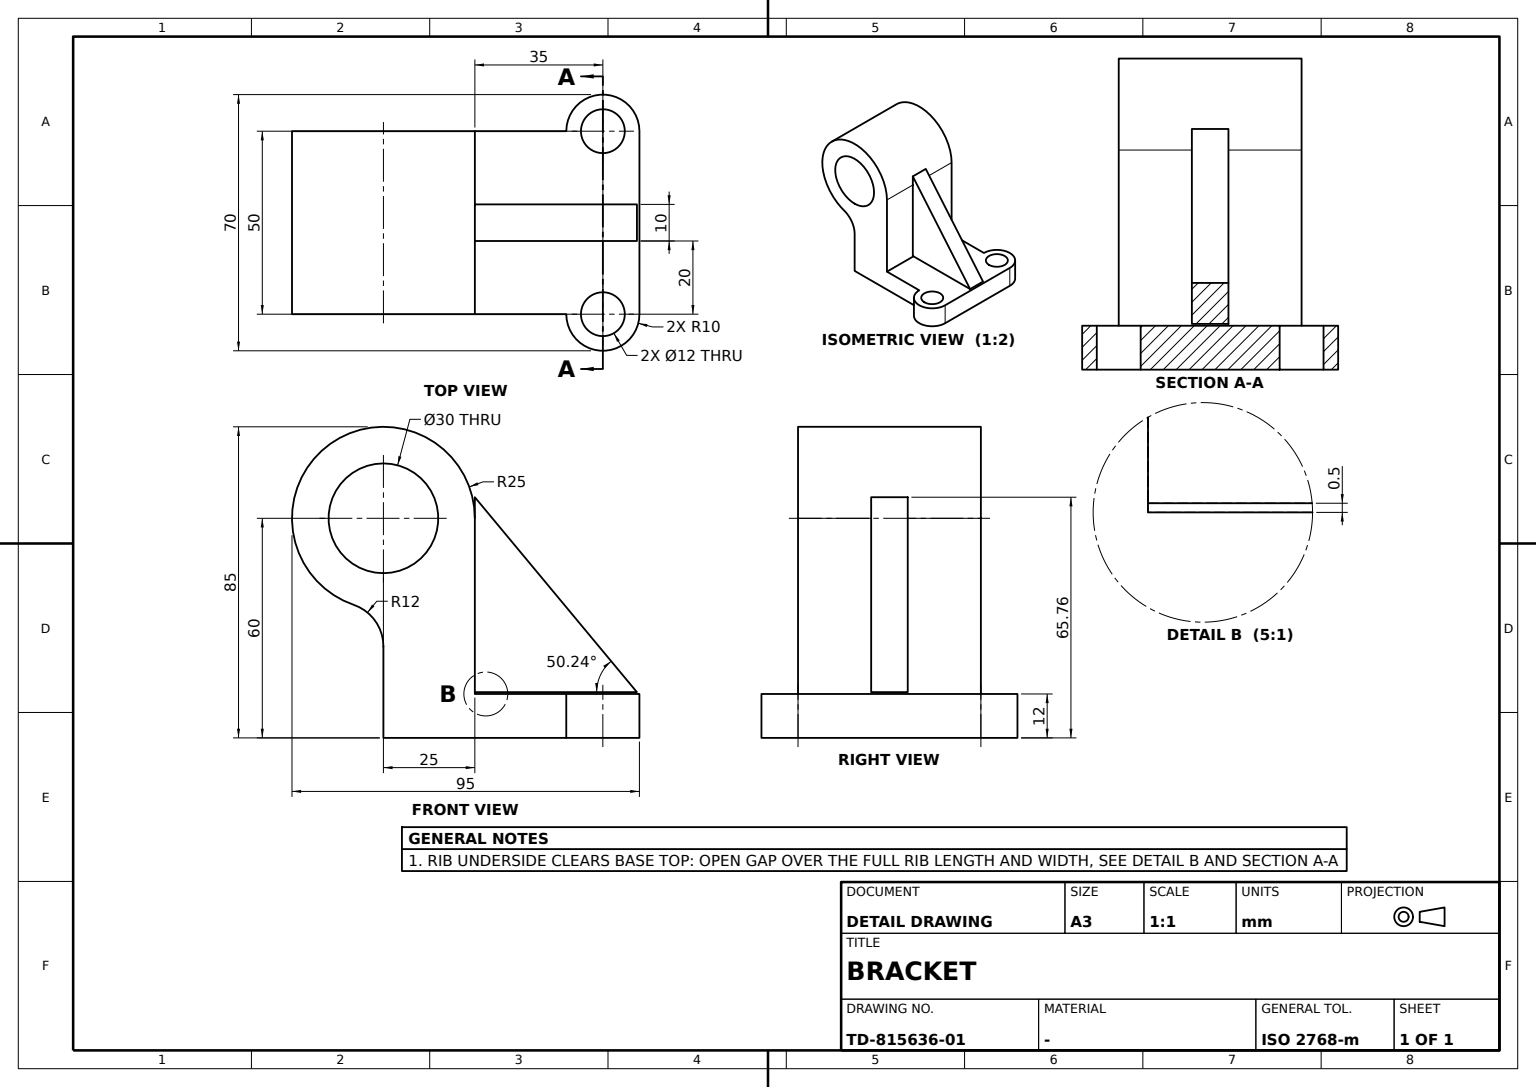
ISO-10303-21;
HEADER;
FILE_DESCRIPTION((''),'2;1');
FILE_NAME('','',(''),(''),'','','');
FILE_SCHEMA(('AUTOMOTIVE_DESIGN'));
ENDSEC;
DATA;
#1=APPLICATION_CONTEXT('');
#2=PRODUCT_CONTEXT('',#1,'mechanical');
#3=PRODUCT('','','',(#2));
#4=PRODUCT_DEFINITION_FORMATION('','',#3);
#5=PRODUCT_DEFINITION_CONTEXT('',#1,'design');
#6=PRODUCT_DEFINITION('','',#4,#5);
#7=PRODUCT_DEFINITION_SHAPE('','',#6);
#8=(LENGTH_UNIT()NAMED_UNIT(*)SI_UNIT(.MILLI.,.METRE.));
#9=(NAMED_UNIT(*)PLANE_ANGLE_UNIT()SI_UNIT($,.RADIAN.));
#10=(NAMED_UNIT(*)SI_UNIT($,.STERADIAN.)SOLID_ANGLE_UNIT());
#11=UNCERTAINTY_MEASURE_WITH_UNIT(LENGTH_MEASURE(0.005),#8,'distance_accuracy_value','');
#12=(GEOMETRIC_REPRESENTATION_CONTEXT(3)GLOBAL_UNCERTAINTY_ASSIGNED_CONTEXT((#11))GLOBAL_UNIT_ASSIGNED_CONTEXT((#8,#9,#10))REPRESENTATION_CONTEXT('',''));
#13=CARTESIAN_POINT('',(20.,0.,6.5));
#14=VERTEX_POINT('',#13);
#15=CARTESIAN_POINT('',(20.,44.314968,6.5));
#16=VERTEX_POINT('',#15);
#17=DIRECTION('',(0.,1.,0.));
#18=VECTOR('',#17,1000.);
#19=LINE('',#13,#18);
#20=EDGE_CURVE('',#14,#16,#19,.T.);
#21=ORIENTED_EDGE('',*,*,#20,.F.);
#22=CARTESIAN_POINT('',(20.,0.,54.));
#23=VERTEX_POINT('',#22);
#24=CARTESIAN_POINT('',(20.,0.,0.));
#25=DIRECTION('',(0.,0.,-1.));
#26=VECTOR('',#25,1000.);
#27=LINE('',#24,#26);
#28=EDGE_CURVE('',#23,#14,#27,.T.);
#29=ORIENTED_EDGE('',*,*,#28,.F.);
#30=CARTESIAN_POINT('',(20.,0.,59.759468));
#31=VERTEX_POINT('',#30);
#32=EDGE_CURVE('',#31,#23,#27,.T.);
#33=ORIENTED_EDGE('',*,*,#32,.F.);
#34=CARTESIAN_POINT('',(20.,29.381753,24.447324));
#35=DIRECTION('',(0.,-0.639605663,0.768703191));
#36=VECTOR('',#35,1000.);
#37=LINE('',#34,#36);
#38=EDGE_CURVE('',#16,#31,#37,.T.);
#39=ORIENTED_EDGE('',*,*,#38,.F.);
#40=EDGE_LOOP('',(#21,#29,#33,#39));
#41=FACE_BOUND('',#40,.T.);
#42=DIRECTION('',(1.,0.,0.));
#43=AXIS2_PLACEMENT_3D('',#24,#42,#17);
#44=PLANE('',#43);
#45=ADVANCED_FACE('',(#41),#44,.F.);
#46=CARTESIAN_POINT('',(0.,-25.,39.));
#47=VERTEX_POINT('',#46);
#48=CARTESIAN_POINT('',(0.,-25.,54.));
#49=AXIS2_PLACEMENT_3D('',#48,#42,#25);
#50=CIRCLE('',#49,15.);
#51=EDGE_CURVE('',#47,#47,#50,.T.);
#52=ORIENTED_EDGE('',*,*,#51,.T.);
#53=EDGE_LOOP('',(#52));
#54=FACE_BOUND('',#53,.T.);
#55=CARTESIAN_POINT('',(0.,-25.,19.));
#56=VERTEX_POINT('',#55);
#57=CARTESIAN_POINT('',(0.,-33.108108,30.351351));
#58=VERTEX_POINT('',#57);
#59=CARTESIAN_POINT('',(0.,-37.,19.));
#60=AXIS2_PLACEMENT_3D('',#59,#42,#25);
#61=CIRCLE('',#60,12.);
#62=EDGE_CURVE('',#56,#58,#61,.T.);
#63=ORIENTED_EDGE('',*,*,#62,.T.);
#64=CARTESIAN_POINT('',(0.,0.,54.));
#65=VERTEX_POINT('',#64);
#66=CIRCLE('',#49,25.);
#67=EDGE_CURVE('',#65,#58,#66,.T.);
#68=ORIENTED_EDGE('',*,*,#67,.F.);
#69=CARTESIAN_POINT('',(0.,0.,6.));
#70=VERTEX_POINT('',#69);
#71=CARTESIAN_POINT('',(0.,0.,0.));
#72=LINE('',#71,#26);
#73=EDGE_CURVE('',#65,#70,#72,.T.);
#74=ORIENTED_EDGE('',*,*,#73,.T.);
#75=CARTESIAN_POINT('',(0.,25.,6.));
#76=VERTEX_POINT('',#75);
#77=LINE('',#69,#18);
#78=EDGE_CURVE('',#70,#76,#77,.T.);
#79=ORIENTED_EDGE('',*,*,#78,.T.);
#80=CARTESIAN_POINT('',(0.,25.,-6.));
#81=VERTEX_POINT('',#80);
#82=DIRECTION('',(0.,0.,1.));
#83=VECTOR('',#82,1000.);
#84=LINE('',#80,#83);
#85=EDGE_CURVE('',#81,#76,#84,.T.);
#86=ORIENTED_EDGE('',*,*,#85,.F.);
#87=CARTESIAN_POINT('',(0.,-25.,-6.));
#88=VERTEX_POINT('',#87);
#89=CARTESIAN_POINT('',(0.,0.,-6.));
#90=DIRECTION('',(0.,-1.,0.));
#91=VECTOR('',#90,1000.);
#92=LINE('',#89,#91);
#93=EDGE_CURVE('',#81,#88,#92,.T.);
#94=ORIENTED_EDGE('',*,*,#93,.T.);
#95=CARTESIAN_POINT('',(0.,-25.,0.));
#96=LINE('',#95,#83);
#97=EDGE_CURVE('',#88,#56,#96,.T.);
#98=ORIENTED_EDGE('',*,*,#97,.T.);
#99=EDGE_LOOP('',(#63,#68,#74,#79,#86,#94,#98));
#100=FACE_BOUND('',#99,.T.);
#101=AXIS2_PLACEMENT_3D('',#71,#42,#17);
#102=PLANE('',#101);
#103=ADVANCED_FACE('',(#54,#100),#102,.F.);
#104=CARTESIAN_POINT('',(50.,-25.,39.));
#105=VERTEX_POINT('',#104);
#106=CARTESIAN_POINT('',(50.,-25.,54.));
#107=AXIS2_PLACEMENT_3D('',#106,#42,#25);
#108=CIRCLE('',#107,15.);
#109=EDGE_CURVE('',#105,#105,#108,.T.);
#110=ORIENTED_EDGE('',*,*,#109,.T.);
#111=EDGE_LOOP('',(#110));
#112=FACE_BOUND('',#111,.T.);
#113=ORIENTED_EDGE('',*,*,#51,.F.);
#114=EDGE_LOOP('',(#113));
#115=FACE_BOUND('',#114,.T.);
#116=CARTESIAN_POINT('',(25.,-25.,54.));
#117=AXIS2_PLACEMENT_3D('',#116,#42,#17);
#118=CYLINDRICAL_SURFACE('',#117,15.);
#119=ADVANCED_FACE('',(#112,#115),#118,.F.);
#120=CARTESIAN_POINT('',(6.,35.,-6.));
#121=VERTEX_POINT('',#120);
#122=CARTESIAN_POINT('',(0.,35.,-6.));
#123=AXIS2_PLACEMENT_3D('',#122,#82,#42);
#124=CIRCLE('',#123,6.);
#125=EDGE_CURVE('',#121,#121,#124,.T.);
#126=ORIENTED_EDGE('',*,*,#125,.F.);
#127=EDGE_LOOP('',(#126));
#128=FACE_BOUND('',#127,.T.);
#129=CARTESIAN_POINT('',(-6.,35.,6.));
#130=VERTEX_POINT('',#129);
#131=CARTESIAN_POINT('',(0.,35.,6.));
#132=DIRECTION('',(-1.,0.,0.));
#133=AXIS2_PLACEMENT_3D('',#131,#25,#132);
#134=CIRCLE('',#133,6.);
#135=EDGE_CURVE('',#130,#130,#134,.F.);
#136=ORIENTED_EDGE('',*,*,#135,.T.);
#137=EDGE_LOOP('',(#136));
#138=FACE_BOUND('',#137,.T.);
#139=CARTESIAN_POINT('',(0.,35.,0.));
#140=AXIS2_PLACEMENT_3D('',#139,#82,#42);
#141=CYLINDRICAL_SURFACE('',#140,6.);
#142=ADVANCED_FACE('',(#128,#138),#141,.F.);
#143=CARTESIAN_POINT('',(50.,-25.,19.));
#144=VERTEX_POINT('',#143);
#145=CARTESIAN_POINT('',(50.,-33.108108,30.351351));
#146=VERTEX_POINT('',#145);
#147=CARTESIAN_POINT('',(50.,-37.,19.));
#148=AXIS2_PLACEMENT_3D('',#147,#42,#25);
#149=CIRCLE('',#148,12.);
#150=EDGE_CURVE('',#144,#146,#149,.T.);
#151=ORIENTED_EDGE('',*,*,#150,.T.);
#152=CARTESIAN_POINT('',(25.,-33.108108,30.351351));
#153=VECTOR('',#42,1000.);
#154=LINE('',#152,#153);
#155=EDGE_CURVE('',#58,#146,#154,.T.);
#156=ORIENTED_EDGE('',*,*,#155,.F.);
#157=ORIENTED_EDGE('',*,*,#62,.F.);
#158=CARTESIAN_POINT('',(25.,-25.,19.));
#159=LINE('',#158,#153);
#160=EDGE_CURVE('',#56,#144,#159,.T.);
#161=ORIENTED_EDGE('',*,*,#160,.T.);
#162=EDGE_LOOP('',(#151,#156,#157,#161));
#163=FACE_BOUND('',#162,.T.);
#164=CARTESIAN_POINT('',(25.,-37.,19.));
#165=AXIS2_PLACEMENT_3D('',#164,#42,#17);
#166=CYLINDRICAL_SURFACE('',#165,12.);
#167=ADVANCED_FACE('',(#163),#166,.F.);
#168=CARTESIAN_POINT('',(30.,44.314968,6.5));
#169=VERTEX_POINT('',#168);
#170=CARTESIAN_POINT('',(30.,0.,59.759468));
#171=VERTEX_POINT('',#170);
#172=CARTESIAN_POINT('',(30.,29.381753,24.447324));
#173=LINE('',#172,#36);
#174=EDGE_CURVE('',#169,#171,#173,.T.);
#175=ORIENTED_EDGE('',*,*,#174,.T.);
#176=CARTESIAN_POINT('',(30.,0.,54.));
#177=VERTEX_POINT('',#176);
#178=CARTESIAN_POINT('',(30.,0.,0.));
#179=LINE('',#178,#26);
#180=EDGE_CURVE('',#171,#177,#179,.T.);
#181=ORIENTED_EDGE('',*,*,#180,.T.);
#182=CARTESIAN_POINT('',(30.,0.,6.5));
#183=VERTEX_POINT('',#182);
#184=EDGE_CURVE('',#177,#183,#179,.T.);
#185=ORIENTED_EDGE('',*,*,#184,.T.);
#186=LINE('',#182,#18);
#187=EDGE_CURVE('',#183,#169,#186,.T.);
#188=ORIENTED_EDGE('',*,*,#187,.T.);
#189=EDGE_LOOP('',(#175,#181,#185,#188));
#190=FACE_BOUND('',#189,.T.);
#191=AXIS2_PLACEMENT_3D('',#178,#42,#17);
#192=PLANE('',#191);
#193=ADVANCED_FACE('',(#190),#192,.T.);
#194=CARTESIAN_POINT('',(44.,35.,6.));
#195=VERTEX_POINT('',#194);
#196=CARTESIAN_POINT('',(50.,35.,6.));
#197=AXIS2_PLACEMENT_3D('',#196,#25,#132);
#198=CIRCLE('',#197,6.);
#199=EDGE_CURVE('',#195,#195,#198,.F.);
#200=ORIENTED_EDGE('',*,*,#199,.T.);
#201=EDGE_LOOP('',(#200));
#202=FACE_BOUND('',#201,.T.);
#203=CARTESIAN_POINT('',(56.,35.,-6.));
#204=VERTEX_POINT('',#203);
#205=CARTESIAN_POINT('',(50.,35.,-6.));
#206=AXIS2_PLACEMENT_3D('',#205,#82,#42);
#207=CIRCLE('',#206,6.);
#208=EDGE_CURVE('',#204,#204,#207,.T.);
#209=ORIENTED_EDGE('',*,*,#208,.F.);
#210=EDGE_LOOP('',(#209));
#211=FACE_BOUND('',#210,.T.);
#212=CARTESIAN_POINT('',(50.,35.,0.));
#213=AXIS2_PLACEMENT_3D('',#212,#82,#42);
#214=CYLINDRICAL_SURFACE('',#213,6.);
#215=ADVANCED_FACE('',(#202,#211),#214,.F.);
#216=CARTESIAN_POINT('',(25.,44.314968,6.5));
#217=LINE('',#216,#153);
#218=EDGE_CURVE('',#16,#169,#217,.T.);
#219=ORIENTED_EDGE('',*,*,#218,.F.);
#220=ORIENTED_EDGE('',*,*,#38,.T.);
#221=CARTESIAN_POINT('',(25.,0.,59.759468));
#222=LINE('',#221,#153);
#223=EDGE_CURVE('',#31,#171,#222,.T.);
#224=ORIENTED_EDGE('',*,*,#223,.T.);
#225=ORIENTED_EDGE('',*,*,#174,.F.);
#226=EDGE_LOOP('',(#219,#220,#224,#225));
#227=FACE_BOUND('',#226,.T.);
#228=DIRECTION('',(0.,0.768703191,0.639605663));
#229=AXIS2_PLACEMENT_3D('',#216,#228,#35);
#230=PLANE('',#229);
#231=ADVANCED_FACE('',(#227),#230,.T.);
#232=CARTESIAN_POINT('',(50.,25.,-6.));
#233=VERTEX_POINT('',#232);
#234=CARTESIAN_POINT('',(50.,45.,-6.));
#235=VERTEX_POINT('',#234);
#236=CIRCLE('',#206,10.);
#237=EDGE_CURVE('',#233,#235,#236,.T.);
#238=ORIENTED_EDGE('',*,*,#237,.T.);
#239=CARTESIAN_POINT('',(50.,45.,6.));
#240=VERTEX_POINT('',#239);
#241=CARTESIAN_POINT('',(50.,45.,0.));
#242=LINE('',#241,#83);
#243=EDGE_CURVE('',#240,#235,#242,.F.);
#244=ORIENTED_EDGE('',*,*,#243,.F.);
#245=CARTESIAN_POINT('',(50.,25.,6.));
#246=VERTEX_POINT('',#245);
#247=CIRCLE('',#197,10.);
#248=EDGE_CURVE('',#246,#240,#247,.F.);
#249=ORIENTED_EDGE('',*,*,#248,.F.);
#250=LINE('',#232,#83);
#251=EDGE_CURVE('',#233,#246,#250,.T.);
#252=ORIENTED_EDGE('',*,*,#251,.F.);
#253=EDGE_LOOP('',(#238,#244,#249,#252));
#254=FACE_BOUND('',#253,.T.);
#255=CYLINDRICAL_SURFACE('',#213,10.);
#256=ADVANCED_FACE('',(#254),#255,.T.);
#257=ORIENTED_EDGE('',*,*,#160,.F.);
#258=ORIENTED_EDGE('',*,*,#97,.F.);
#259=CARTESIAN_POINT('',(50.,-25.,-6.));
#260=VERTEX_POINT('',#259);
#261=LINE('',#87,#153);
#262=EDGE_CURVE('',#88,#260,#261,.T.);
#263=ORIENTED_EDGE('',*,*,#262,.T.);
#264=CARTESIAN_POINT('',(50.,-25.,0.));
#265=LINE('',#264,#83);
#266=EDGE_CURVE('',#260,#144,#265,.T.);
#267=ORIENTED_EDGE('',*,*,#266,.T.);
#268=EDGE_LOOP('',(#257,#258,#263,#267));
#269=FACE_BOUND('',#268,.T.);
#270=AXIS2_PLACEMENT_3D('',#87,#17,#82);
#271=PLANE('',#270);
#272=ADVANCED_FACE('',(#269),#271,.F.);
#273=ORIENTED_EDGE('',*,*,#184,.F.);
#274=CARTESIAN_POINT('',(50.,0.,54.));
#275=VERTEX_POINT('',#274);
#276=CARTESIAN_POINT('',(25.,0.,54.));
#277=LINE('',#276,#153);
#278=EDGE_CURVE('',#177,#275,#277,.T.);
#279=ORIENTED_EDGE('',*,*,#278,.T.);
#280=CARTESIAN_POINT('',(50.,0.,6.));
#281=VERTEX_POINT('',#280);
#282=CARTESIAN_POINT('',(50.,0.,0.));
#283=LINE('',#282,#26);
#284=EDGE_CURVE('',#275,#281,#283,.T.);
#285=ORIENTED_EDGE('',*,*,#284,.T.);
#286=LINE('',#69,#153);
#287=EDGE_CURVE('',#70,#281,#286,.T.);
#288=ORIENTED_EDGE('',*,*,#287,.F.);
#289=ORIENTED_EDGE('',*,*,#73,.F.);
#290=EDGE_CURVE('',#65,#23,#277,.T.);
#291=ORIENTED_EDGE('',*,*,#290,.T.);
#292=ORIENTED_EDGE('',*,*,#28,.T.);
#293=CARTESIAN_POINT('',(0.,0.,6.5));
#294=LINE('',#293,#153);
#295=EDGE_CURVE('',#14,#183,#294,.T.);
#296=ORIENTED_EDGE('',*,*,#295,.T.);
#297=EDGE_LOOP('',(#273,#279,#285,#288,#289,#291,#292,#296));
#298=FACE_BOUND('',#297,.T.);
#299=AXIS2_PLACEMENT_3D('',#64,#90,#25);
#300=PLANE('',#299);
#301=ADVANCED_FACE('',(#298),#300,.F.);
#302=CARTESIAN_POINT('',(0.,45.,6.));
#303=VERTEX_POINT('',#302);
#304=CARTESIAN_POINT('',(0.,45.,-6.));
#305=VERTEX_POINT('',#304);
#306=CARTESIAN_POINT('',(0.,45.,0.));
#307=LINE('',#306,#83);
#308=EDGE_CURVE('',#303,#305,#307,.F.);
#309=ORIENTED_EDGE('',*,*,#308,.F.);
#310=LINE('',#302,#153);
#311=EDGE_CURVE('',#303,#240,#310,.T.);
#312=ORIENTED_EDGE('',*,*,#311,.T.);
#313=ORIENTED_EDGE('',*,*,#243,.T.);
#314=LINE('',#304,#153);
#315=EDGE_CURVE('',#305,#235,#314,.T.);
#316=ORIENTED_EDGE('',*,*,#315,.F.);
#317=EDGE_LOOP('',(#309,#312,#313,#316));
#318=FACE_BOUND('',#317,.T.);
#319=AXIS2_PLACEMENT_3D('',#302,#90,#25);
#320=PLANE('',#319);
#321=ADVANCED_FACE('',(#318),#320,.F.);
#322=EDGE_CURVE('',#23,#177,#277,.T.);
#323=ORIENTED_EDGE('',*,*,#322,.F.);
#324=ORIENTED_EDGE('',*,*,#290,.F.);
#325=ORIENTED_EDGE('',*,*,#67,.T.);
#326=ORIENTED_EDGE('',*,*,#155,.T.);
#327=CIRCLE('',#107,25.);
#328=EDGE_CURVE('',#275,#146,#327,.T.);
#329=ORIENTED_EDGE('',*,*,#328,.F.);
#330=ORIENTED_EDGE('',*,*,#278,.F.);
#331=EDGE_LOOP('',(#323,#324,#325,#326,#329,#330));
#332=FACE_BOUND('',#331,.T.);
#333=CYLINDRICAL_SURFACE('',#117,25.);
#334=ADVANCED_FACE('',(#332),#333,.T.);
#335=ORIENTED_EDGE('',*,*,#295,.F.);
#336=ORIENTED_EDGE('',*,*,#20,.T.);
#337=ORIENTED_EDGE('',*,*,#218,.T.);
#338=ORIENTED_EDGE('',*,*,#187,.F.);
#339=EDGE_LOOP('',(#335,#336,#337,#338));
#340=FACE_BOUND('',#339,.T.);
#341=CARTESIAN_POINT('',(25.,0.,6.5));
#342=AXIS2_PLACEMENT_3D('',#341,#25,#17);
#343=PLANE('',#342);
#344=ADVANCED_FACE('',(#340),#343,.T.);
#345=ORIENTED_EDGE('',*,*,#199,.F.);
#346=EDGE_LOOP('',(#345));
#347=FACE_BOUND('',#346,.T.);
#348=LINE('',#280,#18);
#349=EDGE_CURVE('',#281,#246,#348,.T.);
#350=ORIENTED_EDGE('',*,*,#349,.T.);
#351=ORIENTED_EDGE('',*,*,#248,.T.);
#352=ORIENTED_EDGE('',*,*,#311,.F.);
#353=CIRCLE('',#133,10.);
#354=EDGE_CURVE('',#303,#76,#353,.F.);
#355=ORIENTED_EDGE('',*,*,#354,.T.);
#356=ORIENTED_EDGE('',*,*,#78,.F.);
#357=ORIENTED_EDGE('',*,*,#287,.T.);
#358=EDGE_LOOP('',(#350,#351,#352,#355,#356,#357));
#359=FACE_BOUND('',#358,.T.);
#360=ORIENTED_EDGE('',*,*,#135,.F.);
#361=EDGE_LOOP('',(#360));
#362=FACE_BOUND('',#361,.T.);
#363=AXIS2_PLACEMENT_3D('',#69,#25,#17);
#364=PLANE('',#363);
#365=ADVANCED_FACE('',(#347,#359,#362),#364,.F.);
#366=ORIENTED_EDGE('',*,*,#109,.F.);
#367=EDGE_LOOP('',(#366));
#368=FACE_BOUND('',#367,.T.);
#369=ORIENTED_EDGE('',*,*,#150,.F.);
#370=ORIENTED_EDGE('',*,*,#266,.F.);
#371=CARTESIAN_POINT('',(50.,0.,-6.));
#372=LINE('',#371,#91);
#373=EDGE_CURVE('',#233,#260,#372,.T.);
#374=ORIENTED_EDGE('',*,*,#373,.F.);
#375=ORIENTED_EDGE('',*,*,#251,.T.);
#376=ORIENTED_EDGE('',*,*,#349,.F.);
#377=ORIENTED_EDGE('',*,*,#284,.F.);
#378=ORIENTED_EDGE('',*,*,#328,.T.);
#379=EDGE_LOOP('',(#369,#370,#374,#375,#376,#377,#378));
#380=FACE_BOUND('',#379,.T.);
#381=AXIS2_PLACEMENT_3D('',#282,#42,#17);
#382=PLANE('',#381);
#383=ADVANCED_FACE('',(#368,#380),#382,.T.);
#384=ORIENTED_EDGE('',*,*,#354,.F.);
#385=ORIENTED_EDGE('',*,*,#308,.T.);
#386=CIRCLE('',#123,10.);
#387=EDGE_CURVE('',#305,#81,#386,.T.);
#388=ORIENTED_EDGE('',*,*,#387,.T.);
#389=ORIENTED_EDGE('',*,*,#85,.T.);
#390=EDGE_LOOP('',(#384,#385,#388,#389));
#391=FACE_BOUND('',#390,.T.);
#392=CYLINDRICAL_SURFACE('',#140,10.);
#393=ADVANCED_FACE('',(#391),#392,.T.);
#394=ORIENTED_EDGE('',*,*,#208,.T.);
#395=EDGE_LOOP('',(#394));
#396=FACE_BOUND('',#395,.T.);
#397=ORIENTED_EDGE('',*,*,#125,.T.);
#398=EDGE_LOOP('',(#397));
#399=FACE_BOUND('',#398,.T.);
#400=ORIENTED_EDGE('',*,*,#93,.F.);
#401=ORIENTED_EDGE('',*,*,#387,.F.);
#402=ORIENTED_EDGE('',*,*,#315,.T.);
#403=ORIENTED_EDGE('',*,*,#237,.F.);
#404=ORIENTED_EDGE('',*,*,#373,.T.);
#405=ORIENTED_EDGE('',*,*,#262,.F.);
#406=EDGE_LOOP('',(#400,#401,#402,#403,#404,#405));
#407=FACE_BOUND('',#406,.T.);
#408=AXIS2_PLACEMENT_3D('',#304,#82,#90);
#409=PLANE('',#408);
#410=ADVANCED_FACE('',(#396,#399,#407),#409,.F.);
#411=ORIENTED_EDGE('',*,*,#223,.F.);
#412=ORIENTED_EDGE('',*,*,#32,.T.);
#413=ORIENTED_EDGE('',*,*,#322,.T.);
#414=ORIENTED_EDGE('',*,*,#180,.F.);
#415=EDGE_LOOP('',(#411,#412,#413,#414));
#416=FACE_BOUND('',#415,.T.);
#417=ADVANCED_FACE('',(#416),#300,.T.);
#418=CLOSED_SHELL('',(#45,#103,#119,#142,#167,#193,#215,#231,#256,#272,#301,#321,#334,#344,#365,#383,#393,#410,#417));
#419=MANIFOLD_SOLID_BREP('',#418);
#420=ADVANCED_BREP_SHAPE_REPRESENTATION('',(#419),#12);
#421=SHAPE_DEFINITION_REPRESENTATION(#7,#420);
ENDSEC;
END-ISO-10303-21;
